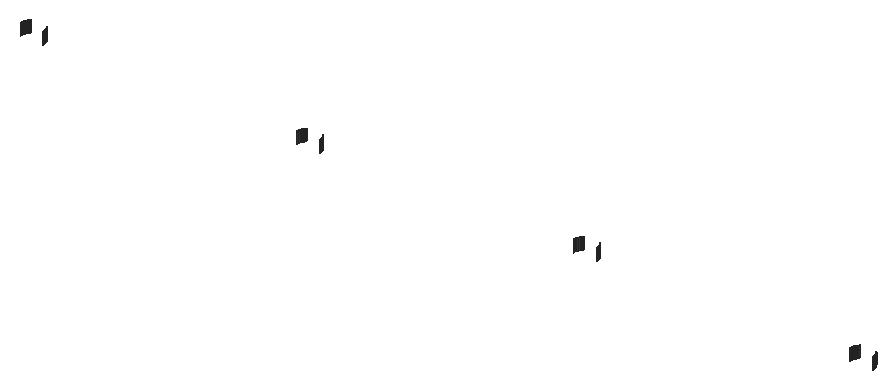
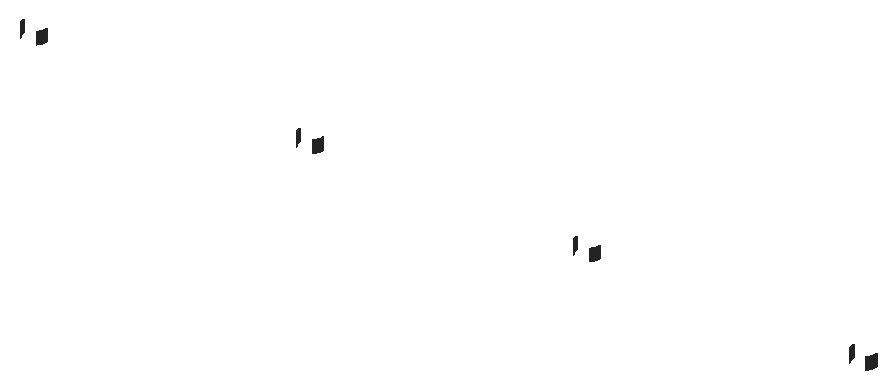
# SketchUp Ruby script. Lengths in inches.
U = 1.inch
M = Sketchup.active_model
def pt(a) = Geom::Point3d.new(a.map { |v| v * U })
def face(e, loops, mat)
  f = e.add_face(loops[0].map { |a| pt(a) })
  loops[1..].each { |l| e.add_face(l.map { |a| pt(a) }).erase! }
  f.material = f.back_material = mat if mat
  f
end
# faces: each face lists its corners as indices into pts; further lists are holes
def faces(e, pts, list, mat = nil) = list.each { |f| face(e, (f[0].is_a?(Array) ? f : [f]).map { |l| l.map { |i| pts[i] } }, mat) }
# xy, xz, yz: faces in a plane at the given z, y or x. An outline is a flat list of corners, or four numbers for a rectangle; further outlines are holes
def ring(l) = l.size == 4 ? [[l[0], l[1]], [l[2], l[1]], [l[2], l[3]], [l[0], l[3]]] : l.each_slice(2).to_a
def flat(e, list, mat, &to3) = list.each { |f| face(e, (f[0].is_a?(Array) ? f : [f]).map { |l| ring(l).map { |u, v| to3.(u, v) } }, mat) }
def xy(e, z, list, mat = nil) = flat(e, list, mat) { |x, y| [x, y, z] }
def xz(e, y, list, mat = nil) = flat(e, list, mat) { |x, z| [x, y, z] }
def yz(e, x, list, mat = nil) = flat(e, list, mat) { |y, z| [x, y, z] }
def lines(e, pts, list) = list.each { |a, b| e.add_line(pt(pts[a]), pt(pts[b])) }
# prism: a flat outline (further loops are holes) pulled along v
def prism(e, loops, v, mat = nil)
  f = face(e, loops, mat); d = Geom::Vector3d.new(v.map { |x| x * U })
  f.pushpull(f.normal.samedirection?(d) ? d.length : -d.length)
end
def box(e, o, s, mat = nil) = prism(e, [[o, [o[0] + s[0], o[1], o[2]], [o[0] + s[0], o[1] + s[1], o[2]], [o[0], o[1] + s[1], o[2]]]], [0, 0, s[2]], mat)
def at(x, y, z, deg = 0) = Geom::Transformation.translation(pt([x, y, z])) * Geom::Transformation.rotation(ORIGIN, Z_AXIS, deg.degrees)
def axes(o, x, y, z) = Geom::Transformation.new([*x, 0, *y, 0, *z, 0, *pt(o).to_a, 1])
def part(name) = M.definitions.add(name)
# library, detail: a bought-in or finely detailed component or shape, given as its bounding box
def library(name, o, s) = part(name).tap { |d| box(d.entities, o, s) }
def detail(e, o, s) = box(e.add_group.entities, o, s)
def put(e, d, t, mat = nil) = e.add_instance(d, t).tap { |i| i.material = mat if mat }
def group(e, t, mat = nil) = e.add_group.tap { |g| g.transformation = t; g.material = mat if mat }.entities
root = M.entities
M.materials.add("1448 AP 8253 RAVEN SONG").color = [64, 64, 63]
yz(root,36.45,[[224.42,372,224.5,375],[224.5,372,224.58,375],[224.58,372,224.66,375]],"1448 AP 8253 RAVEN SONG")
yz(root,42.45,[[224.42,372,224.5,375],[224.5,372,224.58,375],[224.58,372,224.66,375]],"1448 AP 8253 RAVEN SONG")
yz(root,109.03,[[224.42,372,224.5,375],[224.5,372,224.58,375],[224.58,372,224.66,375]],"1448 AP 8253 RAVEN SONG")
yz(root,115.03,[[224.42,372,224.5,375],[224.5,372,224.58,375],[224.58,372,224.66,375]],"1448 AP 8253 RAVEN SONG")
yz(root,181.61,[[224.42,372,224.5,375],[224.5,372,224.58,375],[224.58,372,224.66,375]],"1448 AP 8253 RAVEN SONG")
yz(root,187.61,[[224.5,372,224.58,375],[224.58,372,224.66,375]],"1448 AP 8253 RAVEN SONG")
yz(root,254.19,[[224.5,372,224.58,375],[224.58,372,224.66,375]],"1448 AP 8253 RAVEN SONG")
yz(root,260.1875,[[224.58,372,224.66,375]],"1448 AP 8253 RAVEN SONG")
p = [[260.1875,224.58,372],[260.19,224.5,372],[260.19,224.5,375],[260.1875,224.58,375],[36.45,224.66,372],[36.46,224.74,372],
  [36.46,224.74,375],[36.45,224.66,375],[36.47,224.8125,372],[36.47,224.8125,375],[42.44,224.74,372],[42.45,224.66,372],
  [42.45,224.66,375],[42.44,224.74,375],[42.43,224.8125,372],[42.43,224.8125,375],[109.03,224.66,372],[109.04,224.74,372],
  [109.04,224.74,375],[109.03,224.66,375],[109.05,224.8125,372],[109.05,224.8125,375],[115.02,224.74,372],[115.03,224.66,372],
  [115.03,224.66,375],[115.02,224.74,375],[115.01,224.8125,372],[115.01,224.8125,375],[181.61,224.66,372],[181.62,224.74,372],
  [181.62,224.74,375],[181.61,224.66,375],[181.625,224.8125,372],[181.625,224.8125,375],[187.6,224.74,372],[187.61,224.66,372],
  [187.61,224.66,375],[187.6,224.74,375],[187.59,224.8125,372],[187.59,224.8125,375],[254.19,224.66,372],[254.2,224.74,372],
  [254.2,224.74,375],[254.19,224.66,375],[254.21,224.8125,372],[254.21,224.8125,375],[260.18,224.74,372],[260.1875,224.66,372],
  [260.1875,224.66,375],[260.18,224.74,375],[260.17,224.8125,372],[260.17,224.8125,375],[36.48,224.89,372],[36.48,224.89,375],
  [42.42,224.89,372],[42.42,224.89,375],[109.06,224.89,372],[109.06,224.89,375],[115,224.89,372],[115,224.89,375],
  [181.64,224.89,372],[181.64,224.89,375],[187.58,224.89,372],[187.58,224.89,375],[254.22,224.89,372],[254.22,224.89,375],
  [260.16,224.89,372],[260.16,224.89,375],[36.49,224.97,372],[36.49,224.97,375],[42.41,224.97,372],[42.41,224.97,375],
  [109.07,224.97,372],[109.07,224.97,375],[114.99,224.97,372],[114.99,224.97,375],[181.65,224.97,372],[181.65,224.97,375],
  [187.57,224.97,372],[187.57,224.97,375],[254.23,224.97,372],[254.23,224.97,375],[260.15,224.97,372],[260.15,224.97,375],
  [36.5,225.05,372],[36.5,225.05,375],[36.52,225.125,372],[36.52,225.125,375],[42.4,225.05,372],[42.4,225.05,375],
  [42.38,225.125,372],[42.38,225.125,375],[109.08,225.05,372],[109.08,225.05,375],[109.1,225.125,372],[109.1,225.125,375],
  [114.98,225.05,372],[114.98,225.05,375],[114.96,225.125,372],[114.96,225.125,375],[181.66,225.05,372],[181.66,225.05,375],
  [181.68,225.125,372],[181.68,225.125,375],[187.54,225.125,372],[187.56,225.05,372],[187.56,225.05,375],[187.54,225.125,375],
  [254.24,225.05,372],[254.24,225.05,375],[254.26,225.125,372],[254.26,225.125,375],[260.14,225.05,372],[260.14,225.05,375],
  [260.125,225.125,372],[260.125,225.125,375],[36.53,225.2,372],[36.53,225.2,375],[42.37,225.2,372],[42.37,225.2,375],
  [109.11,225.2,372],[109.11,225.2,375],[114.95,225.2,372],[114.95,225.2,375],[181.69,225.2,372],[181.69,225.2,375],
  [187.53,225.2,372],[187.53,225.2,375],[254.27,225.2,372],[254.27,225.2,375],[260.11,225.2,372],[260.11,225.2,375],
  [36.55,225.28,372],[36.55,225.28,375],[42.35,225.28,372],[42.35,225.28,375],[109.13,225.28,372],[109.13,225.28,375],
  [114.93,225.28,372],[114.93,225.28,375],[181.71,225.28,372],[181.71,225.28,375],[187.51,225.28,372],[187.51,225.28,375],
  [254.29,225.28,372],[254.29,225.28,375],[260.09,225.28,372],[260.09,225.28,375],[36.57,225.35,372],[36.57,225.35,375],
  [42.33,225.35,372],[42.33,225.35,375],[109.15,225.35,372],[109.15,225.35,375],[114.91,225.35,372],[114.91,225.35,375],
  [181.73,225.35,372],[181.73,225.35,375],[187.49,225.35,372],[187.49,225.35,375],[254.3125,225.35,372],[254.3125,225.35,375],
  [260.07,225.35,372],[260.07,225.35,375],[36.6,225.43,372],[36.6,225.43,375],[36.62,225.5,372],[36.62,225.5,375],
  [42.3,225.43,372],[42.3,225.43,375],[42.28,225.5,372],[42.28,225.5,375],[109.18,225.43,372],[109.18,225.43,375],
  [109.2,225.5,372],[109.2,225.5,375],[114.88,225.43,372],[114.88,225.43,375],[114.86,225.5,372],[114.86,225.5,375],
  [181.76,225.43,372],[181.76,225.43,375],[181.78,225.5,372],[181.78,225.5,375],[187.4375,225.5,372],[187.46,225.43,372],
  [187.46,225.43,375],[187.4375,225.5,375],[254.34,225.43,372],[254.34,225.43,375],[254.36,225.5,372],[254.36,225.5,375],
  [260.04,225.43,372],[260.04,225.43,375],[260.02,225.5,372],[260.02,225.5,375],[36.65,225.58,372],[36.65,225.58,375],
  [42.25,225.58,372],[42.25,225.58,375],[109.23,225.58,372],[109.23,225.58,375],[114.83,225.58,372],[114.83,225.58,375],
  [181.81,225.58,372],[181.81,225.58,375],[187.41,225.58,372],[187.41,225.58,375],[254.39,225.58,372],[254.39,225.58,375],
  [259.99,225.58,372],[259.99,225.58,375],[36.68,225.65,372],[36.68,225.65,375],[36.71,225.72,372],[36.71,225.72,375],
  [42.22,225.65,372],[42.22,225.65,375],[42.19,225.72,372],[42.19,225.72,375],[109.26,225.65,372],[109.26,225.65,375],
  [109.29,225.72,372],[109.29,225.72,375],[114.8,225.65,372],[114.8,225.65,375],[114.77,225.72,372],[114.77,225.72,375],
  [181.84,225.65,372],[181.84,225.65,375],[181.87,225.72,372],[181.87,225.72,375],[187.38,225.65,372],[187.38,225.65,375],
  [187.35,225.72,372],[187.35,225.72,375],[254.42,225.65,372],[254.42,225.65,375],[254.45,225.72,372],[254.45,225.72,375],
  [259.93,225.72,372],[259.96,225.65,372],[259.96,225.65,375],[259.93,225.72,375],[36.74,225.79,372],[36.74,225.79,375],
  [42.16,225.79,372],[42.16,225.79,375],[109.32,225.79,372],[109.32,225.79,375],[114.74,225.79,372],[114.74,225.79,375],
  [181.9,225.79,372],[181.9,225.79,375],[187.32,225.79,372],[187.32,225.79,375],[254.48,225.79,372],[254.48,225.79,375],
  [259.9,225.79,372],[259.9,225.79,375],[36.78,225.86,372],[36.78,225.86,375],[42.125,225.86,372],[42.125,225.86,375],
  [109.36,225.86,372],[109.36,225.86,375],[114.7,225.86,372],[114.7,225.86,375],[181.9375,225.86,372],[181.9375,225.86,375],
  [187.28,225.86,372],[187.28,225.86,375],[254.52,225.86,372],[254.52,225.86,375],[259.86,225.86,372],[259.86,225.86,375],
  [36.8125,225.93,372],[36.8125,225.93,375],[36.85,226,372],[36.85,226,375],[42.05,226,372],[42.09,225.93,372],
  [42.09,225.93,375],[42.05,226,375],[109.39,225.93,372],[109.39,225.93,375],[109.43,226,372],[109.43,226,375],
  [114.63,226,372],[114.67,225.93,372],[114.67,225.93,375],[114.63,226,375],[181.97,225.93,372],[181.97,225.93,375],
  [182.01,226,372],[182.01,226,375],[187.25,225.93,372],[187.25,225.93,375],[187.21,226,372],[187.21,226,375],
  [254.55,225.93,372],[254.55,225.93,375],[254.59,226,372],[254.59,226,375],[259.83,225.93,372],[259.83,225.93,375],
  [259.79,226,372],[259.79,226,375],[36.89,226.07,372],[36.89,226.07,375],[42.01,226.07,372],[42.01,226.07,375],
  [109.47,226.07,372],[109.47,226.07,375],[114.59,226.07,372],[114.59,226.07,375],[182.05,226.07,372],[182.05,226.07,375],
  [187.17,226.07,372],[187.17,226.07,375],[254.63,226.07,372],[254.63,226.07,375],[259.75,226.07,372],[259.75,226.07,375],
  [36.93,226.13,372],[36.93,226.13,375],[36.98,226.2,372],[36.98,226.2,375],[41.92,226.2,372],[41.97,226.13,372],
  [41.97,226.13,375],[41.92,226.2,375],[109.51,226.13,372],[109.51,226.13,375],[109.56,226.2,372],[109.56,226.2,375],
  [114.55,226.13,372],[114.55,226.13,375],[114.5,226.2,372],[114.5,226.2,375],[182.09,226.13,372],[182.09,226.13,375],
  [182.14,226.2,372],[182.14,226.2,375],[187.125,226.13,372],[187.125,226.13,375],[187.08,226.2,372],[187.08,226.2,375],
  [254.67,226.13,372],[254.67,226.13,375],[254.72,226.2,372],[254.72,226.2,375],[259.71,226.13,372],[259.71,226.13,375],
  [259.66,226.2,372],[259.66,226.2,375],[37.02,226.26,372],[37.02,226.26,375],[41.88,226.26,372],[41.88,226.26,375],
  [109.6,226.26,372],[109.6,226.26,375],[114.46,226.26,372],[114.46,226.26,375],[182.18,226.26,372],[182.18,226.26,375],
  [187.04,226.26,372],[187.04,226.26,375],[254.76,226.26,372],[254.76,226.26,375],[259.62,226.26,372],[259.62,226.26,375],
  [37.07,226.33,372],[37.07,226.33,375],[37.12,226.39,372],[37.12,226.39,375],[41.83,226.33,372],[41.83,226.33,375],
  [41.78,226.39,372],[41.78,226.39,375],[109.65,226.33,372],[109.65,226.33,375],[109.7,226.39,372],[109.7,226.39,375],
  [114.41,226.33,372],[114.41,226.33,375],[114.36,226.39,372],[114.36,226.39,375],[182.23,226.33,372],[182.23,226.33,375],
  [182.28,226.39,372],[182.28,226.39,375],[186.94,226.39,372],[186.99,226.33,372],[186.99,226.33,375],[186.94,226.39,375],
  [254.81,226.33,372],[254.81,226.33,375],[254.86,226.39,372],[254.86,226.39,375],[259.52,226.39,372],[259.57,226.33,372],
  [259.57,226.33,375],[259.52,226.39,375],[37.17,226.45,372],[37.17,226.45,375],[37.22,226.51,372],[37.22,226.51,375],
  [41.73,226.45,372],[41.73,226.45,375],[41.68,226.51,372],[41.68,226.51,375],[109.75,226.45,372],[109.75,226.45,375],
  [109.8,226.51,372],[109.8,226.51,375],[114.3125,226.45,372],[114.3125,226.45,375],[114.26,226.51,372],[114.26,226.51,375],
  [182.33,226.45,372],[182.33,226.45,375],[182.38,226.51,372],[182.38,226.51,375],[186.84,226.51,372],[186.89,226.45,372],
  [186.89,226.45,375],[186.84,226.51,375],[254.91,226.45,372],[254.91,226.45,375],[254.96,226.51,372],[254.96,226.51,375],
  [259.42,226.51,372],[259.47,226.45,372],[259.47,226.45,375],[259.42,226.51,375],[37.27,226.57,372],[37.27,226.57,375],
  [41.625,226.57,372],[41.625,226.57,375],[109.85,226.57,372],[109.85,226.57,375],[114.21,226.57,372],[114.21,226.57,375],
  [182.43,226.57,372],[182.43,226.57,375],[186.79,226.57,372],[186.79,226.57,375],[255.01,226.57,372],[255.01,226.57,375],
  [259.37,226.57,372],[259.37,226.57,375],[37.33,226.62,372],[37.33,226.62,375],[109.91,226.62,372],[109.91,226.62,375],
  [114.15,226.62,372],[114.15,226.62,375],[182.49,226.62,372],[182.49,226.62,375],[186.73,226.62,372],[186.73,226.62,375],
  [255.07,226.62,372],[255.07,226.62,375],[259.3125,226.62,372],[259.3125,226.62,375]]
faces(root,p,[[0,1,2,3],[4,5,6,7],[5,8,9,6],[10,11,12,13],[14,10,13,15],[16,17,18,19],[17,20,21,18],[22,23,24,25],
  [26,22,25,27],[28,29,30,31],[29,32,33,30],[34,35,36,37],[38,34,37,39],[40,41,42,43],[41,44,45,42],[46,47,48,49],
  [50,46,49,51],[8,52,53,9],[54,14,15,55],[20,56,57,21],[58,26,27,59],[32,60,61,33],[62,38,39,63],[44,64,65,45],
  [66,50,51,67],[52,68,69,53],[70,54,55,71],[56,72,73,57],[74,58,59,75],[60,76,77,61],[78,62,63,79],[64,80,81,65],
  [82,66,67,83],[68,84,85,69],[84,86,87,85],[88,70,71,89],[90,88,89,91],[72,92,93,73],[92,94,95,93],[96,74,75,97],
  [98,96,97,99],[76,100,101,77],[100,102,103,101],[104,105,106,107],[105,78,79,106],[80,108,109,81],[108,110,111,109],[112,82,83,113],
  [114,112,113,115],[86,116,117,87],[118,90,91,119],[94,120,121,95],[122,98,99,123],[102,124,125,103],[126,104,107,127],[110,128,129,111],
  [130,114,115,131],[116,132,133,117],[134,118,119,135],[120,136,137,121],[138,122,123,139],[124,140,141,125],[142,126,127,143],[128,144,145,129],
  [146,130,131,147],[132,148,149,133],[150,134,135,151],[136,152,153,137],[154,138,139,155],[140,156,157,141],[158,142,143,159],[144,160,161,145],
  [162,146,147,163],[148,164,165,149],[164,166,167,165],[168,150,151,169],[170,168,169,171],[152,172,173,153],[172,174,175,173],[176,154,155,177],
  [178,176,177,179],[156,180,181,157],[180,182,183,181],[184,185,186,187],[185,158,159,186],[160,188,189,161],[188,190,191,189],[192,162,163,193],
  [194,192,193,195],[166,196,197,167],[198,170,171,199],[174,200,201,175],[202,178,179,203],[182,204,205,183],[206,184,187,207],[190,208,209,191],
  [210,194,195,211],[196,212,213,197],[212,214,215,213],[216,198,199,217],[218,216,217,219],[200,220,221,201],[220,222,223,221],[224,202,203,225],
  [226,224,225,227],[204,228,229,205],[228,230,231,229],[232,206,207,233],[234,232,233,235],[208,236,237,209],[236,238,239,237],[240,241,242,243],
  [241,210,211,242],[214,244,245,215],[246,218,219,247],[222,248,249,223],[250,226,227,251],[230,252,253,231],[254,234,235,255],[238,256,257,239],
  [258,240,243,259],[244,260,261,245],[262,246,247,263],[248,264,265,249],[266,250,251,267],[252,268,269,253],[270,254,255,271],[256,272,273,257],
  [274,258,259,275],[260,276,277,261],[276,278,279,277],[280,281,282,283],[281,262,263,282],[264,284,285,265],[284,286,287,285],[288,289,290,291],
  [289,266,267,290],[268,292,293,269],[292,294,295,293],[296,270,271,297],[298,296,297,299],[272,300,301,273],[300,302,303,301],[304,274,275,305],
  [306,304,305,307],[278,308,309,279],[310,280,283,311],[286,312,313,287],[314,288,291,315],[294,316,317,295],[318,298,299,319],[302,320,321,303],
  [322,306,307,323],[308,324,325,309],[324,326,327,325],[328,329,330,331],[329,310,311,330],[312,332,333,313],[332,334,335,333],[336,314,315,337],
  [338,336,337,339],[316,340,341,317],[340,342,343,341],[344,318,319,345],[346,344,345,347],[320,348,349,321],[348,350,351,349],[352,322,323,353],
  [354,352,353,355],[326,356,357,327],[358,328,331,359],[334,360,361,335],[362,338,339,363],[342,364,365,343],[366,346,347,367],[350,368,369,351],
  [370,354,355,371],[356,372,373,357],[372,374,375,373],[376,358,359,377],[378,376,377,379],[360,380,381,361],[380,382,383,381],[384,362,363,385],
  [386,384,385,387],[364,388,389,365],[388,390,391,389],[392,393,394,395],[393,366,367,394],[368,396,397,369],[396,398,399,397],[400,401,402,403],
  [401,370,371,402],[374,404,405,375],[404,406,407,405],[408,378,379,409],[410,408,409,411],[382,412,413,383],[412,414,415,413],[416,386,387,417],
  [418,416,417,419],[390,420,421,391],[420,422,423,421],[424,425,426,427],[425,392,395,426],[398,428,429,399],[428,430,431,429],[432,433,434,435],
  [433,400,403,434],[406,436,437,407],[438,410,411,439],[414,440,441,415],[442,418,419,443],[422,444,445,423],[446,424,427,447],[430,448,449,431],
  [450,432,435,451],[436,452,453,437],[440,454,455,441],[456,442,443,457],[444,458,459,445],[460,446,447,461],[448,462,463,449],[464,450,451,465]],"1448 AP 8253 RAVEN SONG")
